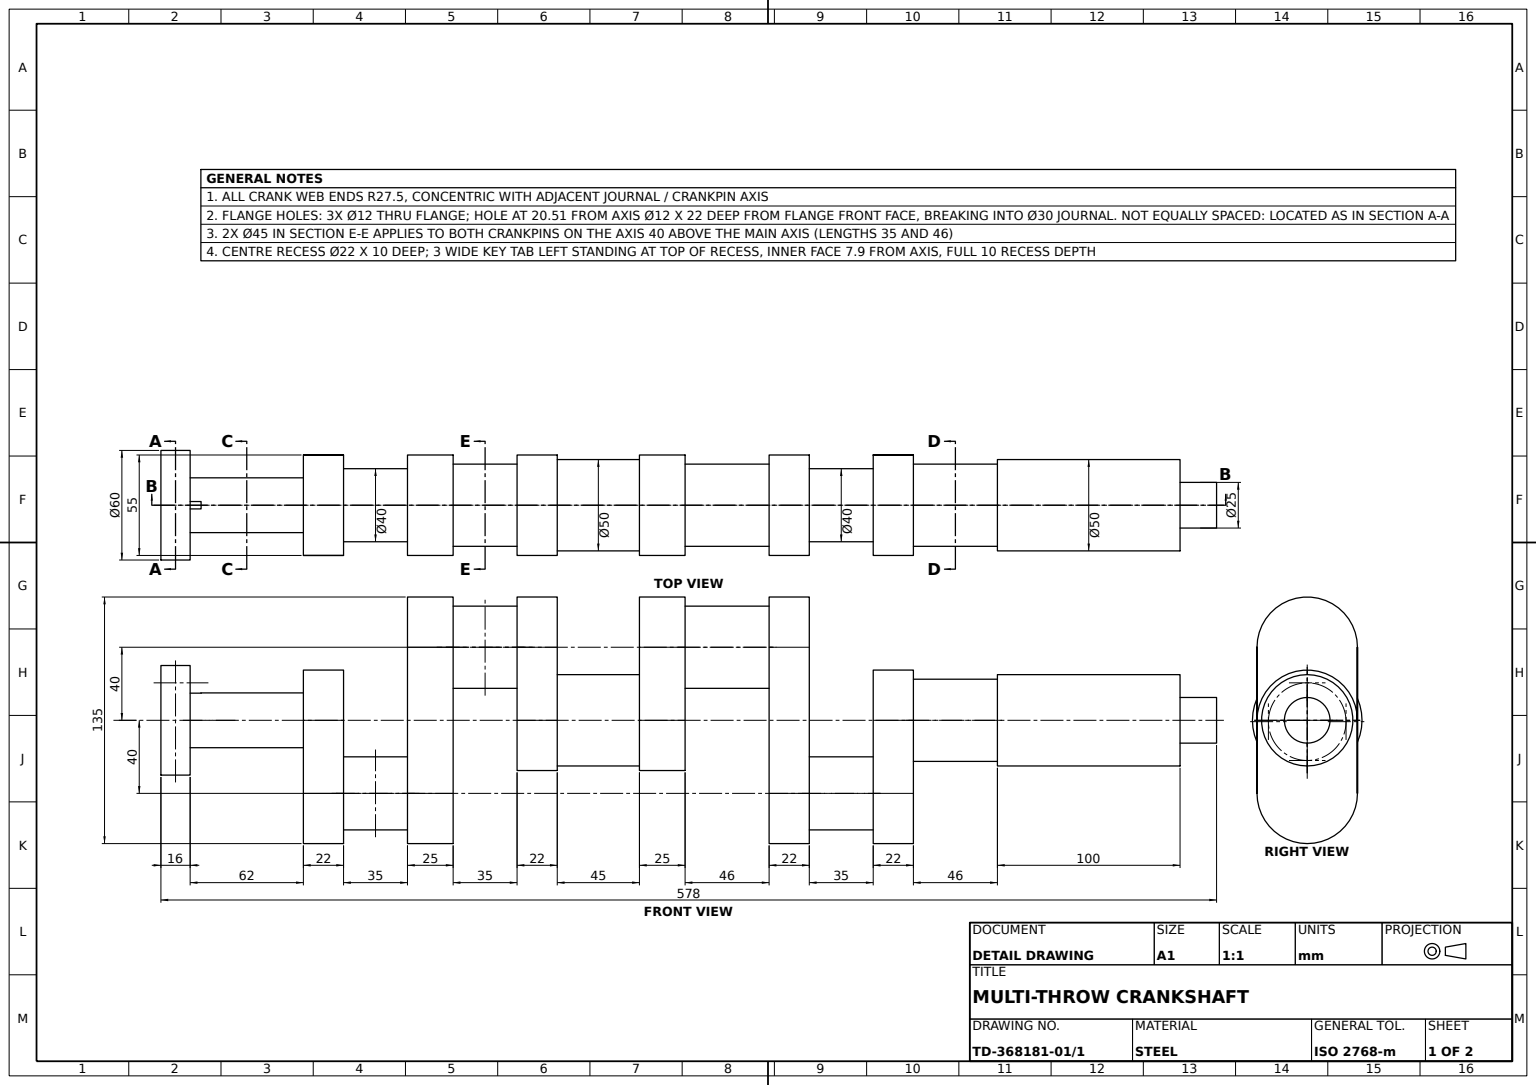
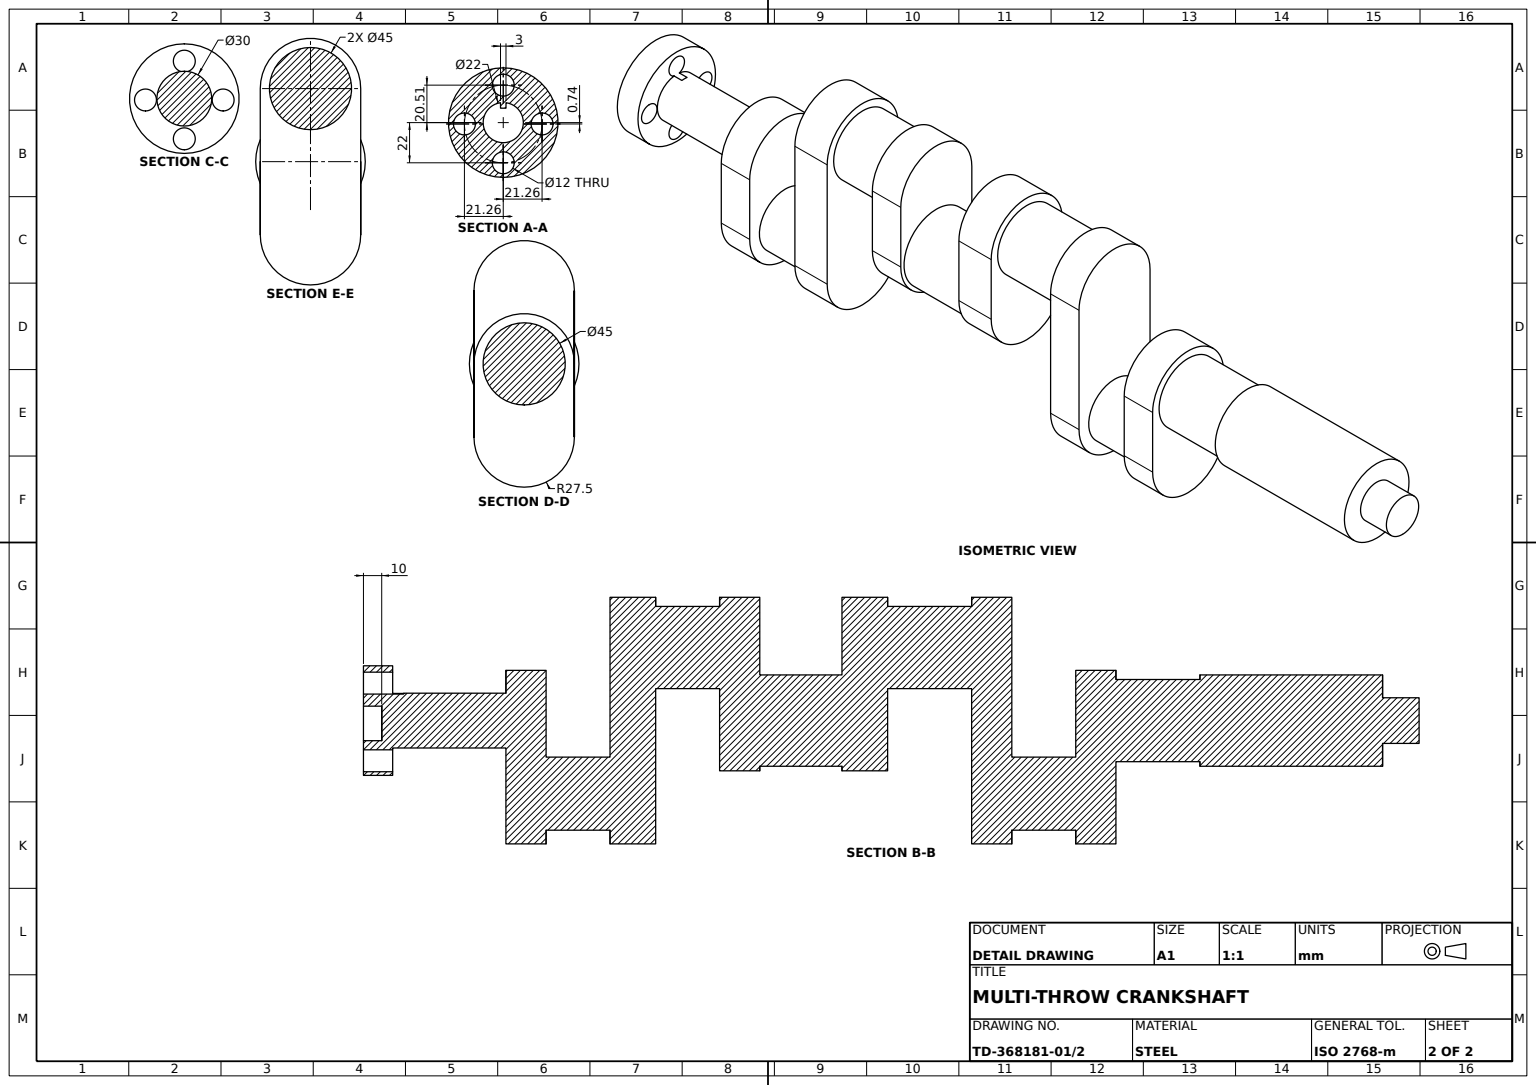
solid
v1 (-40,-27.5,-317)
v2 (-40,27.5,-317)
e1 v1 v2 CIRCLE(AX(P(-40,0,-317),D(0,0,-1),D(-1,0,0)),27.5)
v3 (-40,27.5,-339)
e2 v3 v2 LINE
v4 (-40,-27.5,-339)
e3 v4 v3 CIRCLE(AX(P(-40,0,-339),D(0,0,-1),D(-1,0,0)),27.5)
e4 v4 v1 LINE
face CYL(AX(P(-40,0,-339),D(0,0,1),D(1,0,0)),27.5) [e1 -e2 -e3 e4]
v5 (20,0,-84)
v6 (60,0,-84)
e5 v5 v6 CIRCLE(AX(P(40,0,-84),D(0,0,-1),D(-1,0,0)),20)
e6 v6 v5 CIRCLE(AX(P(40,0,-84),D(0,0,-1),D(-1,0,0)),20)
v7 (0,27.5,-84)
v8 (40,27.5,-84)
e7 v7 v8 LINE
v9 (67.5,0,-84)
e8 v8 v9 CIRCLE(AX(P(40,0,-84),D(0,0,-1),D(-1,0,0)),27.5)
v10 (40,-27.5,-84)
e9 v9 v10 CIRCLE(AX(P(40,0,-84),D(0,0,-1),D(-1,0,0)),27.5)
v11 (0,-27.5,-84)
e10 v10 v11 LINE
e11 v11 v7 CIRCLE(AX(P(0,0,-84),D(0,0,-1),D(-1,0,0)),27.5)
face PLANE(AX(P(0,0,-84),D(0,0,-1),D(-1,0,0))) [-e5 -e6] [e7 e8 e9 e10 e11]
v12 (25,0,-246)
v13 (-25,0,-246)
e12 v12 v13 CIRCLE(AX(P(0,0,-246),D(0,0,-1),D(-1,0,0)),25)
v14 (25,0,-201)
e13 v14 v12 LINE
v15 (-25,0,-201)
e14 v14 v15 CIRCLE(AX(P(0,0,-201),D(0,0,-1),D(-1,0,0)),25)
e15 v15 v13 LINE
face CYL(AX(P(0,0,-261.1485851),D(0,0,-1),D(-1,0,0)),25) [-e12 -e13 e14 e15]
v16 (16,0,0)
v17 (16,0,16)
e16 v16 v17 LINE
v18 (28,0,16)
e17 v17 v18 CIRCLE(AX(P(22,0,16),D(0,0,1),D(1,0,0)),6)
v19 (28,0,0)
e18 v19 v18 LINE
e19 v16 v19 CIRCLE(AX(P(22,0,0),D(0,0,1),D(1,0,0)),6)
face CYL(AX(P(22,0,-6),D(0,0,1),D(1,0,0)),6) rev [e16 e17 -e18 -e19]
v20 (-40,-27.5,-144)
v21 (-40,-27.5,-119)
e20 v20 v21 LINE
v22 (40,-27.5,-144)
e21 v22 v20 LINE
v23 (40,-27.5,-119)
e22 v22 v23 LINE
e23 v23 v21 LINE
face PLANE(AX(P(40,-27.5,-144),D(0,1,0),D(0,0,1))) rev [-e20 -e21 e22 e23]
v24 (25,0,-442)
v25 (-25,0,-442)
e24 v24 v25 CIRCLE(AX(P(0,0,-442),D(0,0,1),D(1,0,0)),25)
e25 v25 v24 CIRCLE(AX(P(0,0,-442),D(0,0,1),D(1,0,0)),25)
v26 (-22.5,0,-442)
v27 (22.5,0,-442)
e26 v26 v27 CIRCLE(AX(P(0,0,-442),D(0,0,1),D(1,0,0)),22.5)
e27 v27 v26 CIRCLE(AX(P(0,0,-442),D(0,0,1),D(1,0,0)),22.5)
face PLANE(AX(P(0,0,-442),D(0,0,1),D(1,0,0))) [e24 e25] [-e26 -e27]
v28 (-40,-27.5,-271)
v29 (-40,-27.5,-246)
e28 v28 v29 LINE
v30 (0,-27.5,-271)
e29 v30 v28 LINE
v31 (0,-27.5,-246)
e30 v30 v31 LINE
e31 v31 v29 LINE
face PLANE(AX(P(0,-27.5,-271),D(0,1,0),D(0,0,1))) rev [-e28 -e29 e30 e31]
v32 (-12.5,0,-562)
v33 (-12.5,0,-542)
e32 v32 v33 LINE
v34 (12.5,0,-562)
e33 v32 v34 CIRCLE(AX(P(0,0,-562),D(0,0,1),D(1,0,0)),12.5)
v35 (12.5,0,-542)
e34 v34 v35 LINE
e35 v33 v35 CIRCLE(AX(P(0,0,-542),D(0,0,1),D(1,0,0)),12.5)
face CYL(AX(P(0,0,-542),D(0,0,1),D(1,0,0)),12.5) [-e32 e33 e34 -e35]
v36 (6.7437452,-21.2562548,0)
v37 (6.7437452,-21.2562548,16)
e36 v36 v37 LINE
v38 (-5.2562548,-21.2562548,16)
e37 v37 v38 CIRCLE(AX(P(0.7437452,-21.2562548,16),D(0,0,1),D(1,0,0)),6)
v39 (-5.2562548,-21.2562548,0)
e38 v39 v38 LINE
e39 v36 v39 CIRCLE(AX(P(0.7437452,-21.2562548,0),D(0,0,1),D(1,0,0)),6)
face CYL(AX(P(0.7437452,-21.2562548,-6),D(0,0,1),D(1,0,0)),6) rev [e36 e37 -e38 -e39]
v40 (-15,0,-6)
v41 (-14.8631996,-2.0212116,-6)
e40 v40 v41 CIRCLE(AX(P(0,0,-6),D(0,0,1),D(1,0,0)),15)
v42 (-15,0,-62)
e41 v40 v42 LINE
v43 (15,0,-62)
e42 v43 v42 CIRCLE(AX(P(0,0,-62),D(0,0,-1),D(-1,0,0)),15)
v44 (15,0,0)
e43 v44 v43 LINE
v45 (-14.8631996,-2.0212116,0)
e44 v44 v45 CIRCLE(AX(P(0,0,0),D(0,0,-1),D(-1,0,0)),15)
e45 v45 v41 LINE
face CYL(AX(P(0,0,-63.5307628),D(0,0,-1),D(-1,0,0)),15) [-e40 e41 -e42 -e43 e44 e45]
e46 v39 v36 CIRCLE(AX(P(0.7437452,-21.2562548,0),D(0,0,1),D(1,0,0)),6)
e47 v38 v37 CIRCLE(AX(P(0.7437452,-21.2562548,16),D(0,0,1),D(1,0,0)),6)
face CYL(AX(P(0.7437452,-21.2562548,-6),D(0,0,1),D(1,0,0)),6) rev [-e46 e38 e47 -e36]
v46 (-26.5125097,0,0)
v47 (-26.5125097,0,16)
e48 v46 v47 LINE
v48 (-14.5125097,0,16)
e49 v47 v48 CIRCLE(AX(P(-20.5125097,0,16),D(0,0,1),D(1,0,0)),6)
v49 (-14.5125097,0,-6)
e50 v49 v48 LINE
e51 v41 v49 CIRCLE(AX(P(-20.5125097,0,-6),D(0,0,1),D(1,0,0)),6)
e52 v46 v45 CIRCLE(AX(P(-20.5125097,0,0),D(0,0,1),D(1,0,0)),6)
face CYL(AX(P(-20.5125097,0,-6),D(0,0,1),D(1,0,0)),6) rev [e48 e49 -e50 -e51 -e45 -e52]
v50 (40,27.5,-317)
v51 (67.5,0,-317)
e53 v50 v51 CIRCLE(AX(P(40,0,-317),D(0,0,-1),D(-1,0,0)),27.5)
v52 (67.5,0,-339)
e54 v52 v51 LINE
v53 (40,27.5,-339)
e55 v53 v52 CIRCLE(AX(P(40,0,-339),D(0,0,-1),D(-1,0,0)),27.5)
e56 v53 v50 LINE
face CYL(AX(P(40,0,-339),D(0,0,1),D(1,0,0)),27.5) [e53 -e54 -e55 e56]
v54 (-7.8972474,1.5,6)
v55 (-7.8972474,1.5,16)
e57 v54 v55 LINE
v56 (-7.8972474,-1.5,16)
e58 v55 v56 LINE
v57 (-7.8972474,-1.5,6)
e59 v57 v56 LINE
e60 v54 v57 LINE
face PLANE(AX(P(-7.8972474,1.5,6),D(-1,0,0),D(0,0,1))) rev [e57 e58 -e59 -e60]
v58 (-10.8972474,-1.5,6)
v59 (-10.8972474,-1.5,16)
e61 v58 v59 LINE
v60 (11,0,16)
e62 v59 v60 CIRCLE(AX(P(0,0,16),D(0,0,1),D(1,0,0)),11)
v61 (11,0,6)
e63 v61 v60 LINE
e64 v58 v61 CIRCLE(AX(P(0,0,6),D(0,0,1),D(1,0,0)),11)
face CYL(AX(P(0,0,6),D(0,0,1),D(1,0,0)),11) rev [e61 e62 -e63 -e64]
v62 (67.5,0,-396)
v63 (40,-27.5,-396)
e65 v62 v63 CIRCLE(AX(P(40,0,-396),D(0,0,-1),D(-1,0,0)),27.5)
v64 (67.5,0,-374)
e66 v62 v64 LINE
v65 (40,-27.5,-374)
e67 v64 v65 CIRCLE(AX(P(40,0,-374),D(0,0,-1),D(-1,0,0)),27.5)
e68 v63 v65 LINE
face CYL(AX(P(40,0,-396),D(0,0,1),D(1,0,0)),27.5) [-e65 e66 e67 -e68]
v66 (0,27.5,-62)
v67 (40,27.5,-62)
e69 v66 v67 LINE
e70 v8 v67 LINE
e71 v7 v66 LINE
face PLANE(AX(P(40,27.5,-84),D(0,-1,0),D(1,0,0))) rev [e69 -e70 -e7 e71]
v68 (20,0,-339)
v69 (60,0,-339)
e72 v68 v69 CIRCLE(AX(P(40,0,-339),D(0,0,-1),D(-1,0,0)),20)
e73 v69 v68 CIRCLE(AX(P(40,0,-339),D(0,0,-1),D(-1,0,0)),20)
e74 v3 v53 LINE
v70 (40,-27.5,-339)
e75 v52 v70 CIRCLE(AX(P(40,0,-339),D(0,0,-1),D(-1,0,0)),27.5)
e76 v70 v4 LINE
face PLANE(AX(P(40,0,-339),D(0,0,-1),D(-1,0,0))) [-e72 -e73] [e74 e55 e75 e76 e3]
v71 (-40,27.5,-144)
v72 (-40,27.5,-119)
e77 v71 v72 LINE
e78 v20 v71 CIRCLE(AX(P(-40,0,-144),D(0,0,-1),D(-1,0,0)),27.5)
e79 v21 v72 CIRCLE(AX(P(-40,0,-119),D(0,0,-1),D(-1,0,0)),27.5)
face CYL(AX(P(-40,0,-144),D(0,0,1),D(1,0,0)),27.5) [-e77 -e78 e20 e79]
e80 v35 v33 CIRCLE(AX(P(0,0,-542),D(0,0,1),D(1,0,0)),12.5)
e81 v34 v32 CIRCLE(AX(P(0,0,-562),D(0,0,1),D(1,0,0)),12.5)
face CYL(AX(P(0,0,-542),D(0,0,1),D(1,0,0)),12.5) [-e80 -e34 e81 e32]
v73 (0,27.5,-271)
v74 (27.5,0,-271)
e82 v73 v74 CIRCLE(AX(P(0,0,-271),D(0,0,-1),D(-1,0,0)),27.5)
e83 v74 v30 CIRCLE(AX(P(0,0,-271),D(0,0,-1),D(-1,0,0)),27.5)
v75 (-40,27.5,-271)
e84 v28 v75 CIRCLE(AX(P(-40,0,-271),D(0,0,-1),D(-1,0,0)),27.5)
e85 v73 v75 LINE
v76 (-17.5,0,-271)
v77 (-62.5,0,-271)
e86 v76 v77 CIRCLE(AX(P(-40,0,-271),D(0,0,-1),D(-1,0,0)),22.5)
e87 v77 v76 CIRCLE(AX(P(-40,0,-271),D(0,0,-1),D(-1,0,0)),22.5)
face PLANE(AX(P(0,0,-271),D(0,0,-1),D(-1,0,0))) [e82 e83 e29 e84 -e85] [-e86 -e87]
v78 (0,-27.5,-396)
v79 (0,-27.5,-374)
e88 v78 v79 LINE
e89 v63 v78 LINE
e90 v65 v79 LINE
face PLANE(AX(P(0,-27.5,-396),D(0,1,0),D(-1,0,0))) rev [-e88 -e89 e68 e90]
v80 (-17.5,0,-317)
e91 v80 v76 LINE
v81 (-62.5,0,-317)
e92 v80 v81 CIRCLE(AX(P(-40,0,-317),D(0,0,1),D(1,0,0)),22.5)
e93 v81 v77 LINE
face CYL(AX(P(-40,0,-271),D(0,0,1),D(1,0,0)),22.5) [e87 -e91 e92 e93]
e94 v19 v16 CIRCLE(AX(P(22,0,0),D(0,0,1),D(1,0,0)),6)
e95 v18 v17 CIRCLE(AX(P(22,0,16),D(0,0,1),D(1,0,0)),6)
face CYL(AX(P(22,0,-6),D(0,0,1),D(1,0,0)),6) rev [-e94 e18 e95 -e16]
v82 (-40,27.5,-246)
e96 v75 v82 LINE
e97 v29 v82 CIRCLE(AX(P(-40,0,-246),D(0,0,-1),D(-1,0,0)),27.5)
face CYL(AX(P(-40,0,-271),D(0,0,1),D(1,0,0)),27.5) [-e96 -e84 e28 e97]
v83 (-10.8972474,1.5,6)
e98 v61 v83 CIRCLE(AX(P(0,0,6),D(0,0,1),D(1,0,0)),11)
v84 (-10.8972474,1.5,16)
e99 v60 v84 CIRCLE(AX(P(0,0,16),D(0,0,1),D(1,0,0)),11)
e100 v83 v84 LINE
face CYL(AX(P(0,0,6),D(0,0,1),D(1,0,0)),11) rev [-e98 e63 e99 -e100]
v85 (-40,27.5,-201)
v86 (0,27.5,-201)
e101 v85 v86 LINE
v87 (-40,27.5,-179)
e102 v85 v87 LINE
v88 (0,27.5,-179)
e103 v87 v88 LINE
e104 v86 v88 LINE
face PLANE(AX(P(0,27.5,-201),D(0,-1,0),D(0,0,-1))) rev [-e101 e102 e103 -e104]
e105 v81 v80 CIRCLE(AX(P(-40,0,-317),D(0,0,1),D(1,0,0)),22.5)
v89 (40,-27.5,-317)
e106 v51 v89 CIRCLE(AX(P(40,0,-317),D(0,0,-1),D(-1,0,0)),27.5)
e107 v2 v50 LINE
e108 v89 v1 LINE
face PLANE(AX(P(40,0,-317),D(0,0,-1),D(-1,0,0))) rev [-e105 -e92] [-e106 -e53 -e107 -e1 -e108]
v90 (25,0,-542)
e109 v90 v24 LINE
v91 (-25,0,-542)
e110 v90 v91 CIRCLE(AX(P(0,0,-542),D(0,0,1),D(1,0,0)),25)
e111 v91 v25 LINE
face CYL(AX(P(0,0,-442),D(0,0,1),D(1,0,0)),25) [-e24 -e109 e110 e111]
e112 v91 v90 CIRCLE(AX(P(0,0,-542),D(0,0,1),D(1,0,0)),25)
face CYL(AX(P(0,0,-442),D(0,0,1),D(1,0,0)),25) [e109 -e25 -e111 e112]
v92 (0,-27.5,-62)
e113 v92 v66 CIRCLE(AX(P(0,0,-62),D(0,0,-1),D(-1,0,0)),27.5)
e114 v11 v92 LINE
face CYL(AX(P(0,0,-84),D(0,0,1),D(1,0,0)),27.5) [e113 -e71 -e11 e114]
v93 (40,-27.5,-62)
e115 v93 v92 LINE
v94 (67.5,0,-62)
e116 v94 v93 CIRCLE(AX(P(40,0,-62),D(0,0,-1),D(-1,0,0)),27.5)
e117 v67 v94 CIRCLE(AX(P(40,0,-62),D(0,0,-1),D(-1,0,0)),27.5)
e118 v42 v43 CIRCLE(AX(P(0,0,-62),D(0,0,-1),D(-1,0,0)),15)
face PLANE(AX(P(0,0,-62),D(0,0,-1),D(-1,0,0))) rev [-e69 -e113 -e115 -e116 -e117] [e118 e42]
face PLANE(AX(P(0,0,-542),D(0,0,-1),D(-1,0,0))) [e80 e35] [-e112 -e110]
e119 v10 v93 LINE
face PLANE(AX(P(40,-27.5,-84),D(0,1,0),D(-1,0,0))) rev [e115 -e114 -e10 e119]
v95 (-14.8631996,2.0212116,0)
e120 v95 v44 CIRCLE(AX(P(0,0,0),D(0,0,-1),D(-1,0,0)),15)
v96 (-14.8631996,2.0212116,-6)
e121 v96 v40 CIRCLE(AX(P(0,0,-6),D(0,0,1),D(1,0,0)),15)
e122 v96 v95 LINE
face CYL(AX(P(0,0,-63.5307628),D(0,0,-1),D(-1,0,0)),15) [e120 e43 -e118 -e41 -e121 e122]
e123 v15 v14 CIRCLE(AX(P(0,0,-201),D(0,0,-1),D(-1,0,0)),25)
v97 (27.5,0,-201)
e124 v86 v97 CIRCLE(AX(P(0,0,-201),D(0,0,-1),D(-1,0,0)),27.5)
v98 (0,-27.5,-201)
e125 v97 v98 CIRCLE(AX(P(0,0,-201),D(0,0,-1),D(-1,0,0)),27.5)
v99 (-40,-27.5,-201)
e126 v98 v99 LINE
e127 v99 v85 CIRCLE(AX(P(-40,0,-201),D(0,0,-1),D(-1,0,0)),27.5)
face PLANE(AX(P(0,0,-201),D(0,0,-1),D(-1,0,0))) [-e14 -e123] [e124 e125 e126 e127 e101]
e128 v83 v54 LINE
e129 v57 v58 LINE
face PLANE(AX(P(0,0,6),D(0,0,1),D(1,0,0))) [e98 e128 e60 e129 e64]
v100 (6.7437452,21.2562548,0)
v101 (-5.2562548,21.2562548,0)
e130 v100 v101 CIRCLE(AX(P(0.7437452,21.2562548,0),D(0,0,1),D(1,0,0)),6)
v102 (6.7437452,21.2562548,16)
e131 v100 v102 LINE
v103 (-5.2562548,21.2562548,16)
e132 v102 v103 CIRCLE(AX(P(0.7437452,21.2562548,16),D(0,0,1),D(1,0,0)),6)
e133 v101 v103 LINE
face CYL(AX(P(0.7437452,21.2562548,-6),D(0,0,1),D(1,0,0)),6) rev [-e130 e131 e132 -e133]
e134 v56 v59 LINE
face PLANE(AX(P(-7.8972474,-1.5,6),D(0,1,0),D(-1,0,0))) rev [e59 e134 -e61 -e129]
v104 (40,27.5,-374)
e135 v104 v64 CIRCLE(AX(P(40,0,-374),D(0,0,-1),D(-1,0,0)),27.5)
v105 (0,27.5,-374)
e136 v104 v105 LINE
e137 v79 v105 CIRCLE(AX(P(0,0,-374),D(0,0,-1),D(-1,0,0)),27.5)
v106 (20,0,-374)
v107 (60,0,-374)
e138 v106 v107 CIRCLE(AX(P(40,0,-374),D(0,0,1),D(1,0,0)),20)
e139 v107 v106 CIRCLE(AX(P(40,0,-374),D(0,0,1),D(1,0,0)),20)
face PLANE(AX(P(0,0,-374),D(0,0,-1),D(-1,0,0))) rev [-e67 -e135 e136 -e137 -e90] [-e138 -e139]
v108 (40,27.5,-144)
e140 v71 v108 LINE
v109 (67.5,0,-144)
e141 v108 v109 CIRCLE(AX(P(40,0,-144),D(0,0,-1),D(-1,0,0)),27.5)
e142 v109 v22 CIRCLE(AX(P(40,0,-144),D(0,0,-1),D(-1,0,0)),27.5)
v110 (-62.5,0,-144)
v111 (-17.5,0,-144)
e143 v110 v111 CIRCLE(AX(P(-40,0,-144),D(0,0,-1),D(-1,0,0)),22.5)
e144 v111 v110 CIRCLE(AX(P(-40,0,-144),D(0,0,-1),D(-1,0,0)),22.5)
face PLANE(AX(P(40,0,-144),D(0,0,-1),D(-1,0,0))) [e21 e78 e140 e141 e142] [-e143 -e144]
v112 (27.5,0,-246)
e145 v74 v112 LINE
e146 v112 v31 CIRCLE(AX(P(0,0,-246),D(0,0,-1),D(-1,0,0)),27.5)
face CYL(AX(P(0,0,-271),D(0,0,1),D(1,0,0)),27.5) [e145 e146 -e30 -e83]
e147 v103 v102 CIRCLE(AX(P(0.7437452,21.2562548,16),D(0,0,1),D(1,0,0)),6)
e148 v101 v100 CIRCLE(AX(P(0.7437452,21.2562548,0),D(0,0,1),D(1,0,0)),6)
face CYL(AX(P(0.7437452,21.2562548,-6),D(0,0,1),D(1,0,0)),6) rev [e133 e147 -e131 -e148]
face PLANE(AX(P(12.5,0,-562),D(0,0,-1),D(-1,0,0))) [-e81 -e33]
e149 v9 v94 LINE
face CYL(AX(P(40,0,-84),D(0,0,1),D(1,0,0)),27.5) [-e149 -e8 e70 e117]
e150 v70 v89 LINE
face CYL(AX(P(40,0,-339),D(0,0,1),D(1,0,0)),27.5) [-e75 e54 e106 -e150]
v113 (-17.5,0,-179)
v114 (-62.5,0,-179)
e151 v113 v114 CIRCLE(AX(P(-40,0,-179),D(0,0,1),D(1,0,0)),22.5)
e152 v114 v110 LINE
e153 v113 v111 LINE
face CYL(AX(P(-40,0,-144),D(0,0,1),D(1,0,0)),22.5) [e151 e152 e143 -e153]
e154 v13 v12 CIRCLE(AX(P(0,0,-246),D(0,0,-1),D(-1,0,0)),25)
face CYL(AX(P(0,0,-261.1485851),D(0,0,-1),D(-1,0,0)),25) [e13 -e154 -e15 e123]
v115 (40,27.5,-396)
e155 v115 v62 CIRCLE(AX(P(40,0,-396),D(0,0,-1),D(-1,0,0)),27.5)
e156 v115 v104 LINE
face CYL(AX(P(40,0,-396),D(0,0,1),D(1,0,0)),27.5) [-e66 -e155 e156 e135]
v116 (-40,-27.5,-179)
e157 v99 v116 LINE
v117 (0,-27.5,-179)
e158 v98 v117 LINE
e159 v117 v116 LINE
face PLANE(AX(P(0,-27.5,-201),D(0,1,0),D(0,0,1))) rev [-e157 -e126 e158 e159]
v118 (27.5,0,-179)
e160 v97 v118 LINE
e161 v118 v117 CIRCLE(AX(P(0,0,-179),D(0,0,-1),D(-1,0,0)),27.5)
face CYL(AX(P(0,0,-201),D(0,0,1),D(1,0,0)),27.5) [-e125 e160 e161 -e158]
v119 (60,0,-119)
e162 v119 v6 LINE
v120 (20,0,-119)
e163 v120 v5 LINE
e164 v120 v119 CIRCLE(AX(P(40,0,-119),D(0,0,1),D(1,0,0)),20)
face CYL(AX(P(40,0,-84),D(0,0,1),D(1,0,0)),20) [e162 e6 -e163 e164]
face CYL(AX(P(-40,0,-271),D(0,0,1),D(1,0,0)),22.5) [e105 e91 e86 -e93]
e165 v116 v87 CIRCLE(AX(P(-40,0,-179),D(0,0,-1),D(-1,0,0)),27.5)
face CYL(AX(P(-40,0,-201),D(0,0,1),D(1,0,0)),27.5) [-e127 e157 e165 -e102]
v121 (40,27.5,-119)
e166 v108 v121 LINE
e167 v72 v121 LINE
face PLANE(AX(P(40,27.5,-144),D(0,-1,0),D(0,0,-1))) rev [-e166 -e140 e77 e167]
v122 (67.5,0,-119)
e168 v122 v23 CIRCLE(AX(P(40,0,-119),D(0,0,-1),D(-1,0,0)),27.5)
e169 v109 v122 LINE
face CYL(AX(P(40,0,-144),D(0,0,1),D(1,0,0)),27.5) [e168 -e22 -e142 e169]
v123 (0,27.5,-246)
e170 v123 v112 CIRCLE(AX(P(0,0,-246),D(0,0,-1),D(-1,0,0)),27.5)
e171 v123 v82 LINE
face PLANE(AX(P(0,0,-246),D(0,0,-1),D(-1,0,0))) rev [e154 e12] [-e31 -e146 -e170 e171 -e97]
v124 (30,0,16)
v125 (-30,0,16)
e172 v124 v125 CIRCLE(AX(P(0,0,16),D(0,0,1),D(1,0,0)),30)
v126 (30,0,0)
e173 v124 v126 LINE
v127 (-30,0,0)
e174 v126 v127 CIRCLE(AX(P(0,0,0),D(0,0,1),D(1,0,0)),30)
e175 v125 v127 LINE
face CYL(AX(P(0,0,16),D(0,0,-1),D(-1,0,0)),30) [-e172 e173 e174 -e175]
e176 v84 v55 LINE
face PLANE(AX(P(-10.8972474,1.5,6),D(0,-1,0),D(1,0,0))) rev [e176 -e57 -e128 e100]
e177 v114 v113 CIRCLE(AX(P(-40,0,-179),D(0,0,1),D(1,0,0)),22.5)
e178 v88 v118 CIRCLE(AX(P(0,0,-179),D(0,0,-1),D(-1,0,0)),27.5)
face PLANE(AX(P(0,0,-179),D(0,0,-1),D(-1,0,0))) rev [-e177 -e151] [-e178 -e103 -e165 -e159 -e161]
e179 v127 v126 CIRCLE(AX(P(0,0,0),D(0,0,1),D(1,0,0)),30)
e180 v95 v46 CIRCLE(AX(P(-20.5125097,0,0),D(0,0,1),D(1,0,0)),6)
face PLANE(AX(P(0,0,0),D(0,0,1),D(1,0,0))) rev [e19 e94] [e39 e46] [e148 e130] [-e174 -e179] [e180 e52 -e44 -e120]
e181 v106 v68 LINE
e182 v107 v69 LINE
face CYL(AX(P(40,0,-339),D(0,0,1),D(1,0,0)),20) [e73 -e181 e138 e182]
face CYL(AX(P(40,0,-84),D(0,0,1),D(1,0,0)),27.5) [-e119 -e9 e149 e116]
e183 v73 v123 LINE
face PLANE(AX(P(0,27.5,-271),D(0,1,0),D(0,0,1))) [e96 -e171 -e183 e85]
e184 v121 v122 CIRCLE(AX(P(40,0,-119),D(0,0,-1),D(-1,0,0)),27.5)
face CYL(AX(P(40,0,-144),D(0,0,1),D(1,0,0)),27.5) [e184 -e169 -e141 e166]
face CYL(AX(P(0,0,-271),D(0,0,1),D(1,0,0)),27.5) [e183 e170 -e145 -e82]
v128 (-22.5,0,-396)
e185 v26 v128 LINE
v129 (22.5,0,-396)
e186 v129 v128 CIRCLE(AX(P(0,0,-396),D(0,0,1),D(1,0,0)),22.5)
e187 v27 v129 LINE
face CYL(AX(P(0,0,-396),D(0,0,1),D(1,0,0)),22.5) [e27 e185 -e186 -e187]
e188 v48 v47 CIRCLE(AX(P(-20.5125097,0,16),D(0,0,1),D(1,0,0)),6)
e189 v125 v124 CIRCLE(AX(P(0,0,16),D(0,0,1),D(1,0,0)),30)
face PLANE(AX(P(0,0,16),D(0,0,1),D(1,0,0))) [-e95 -e17] [-e188 -e49] [-e134 -e58 -e176 -e99 -e62] [-e37 -e47] [e189 e172] [-e132 -e147]
face PLANE(AX(P(40,27.5,-339),D(0,-1,0),D(1,0,0))) rev [-e74 e2 e107 -e56]
v130 (0,27.5,-396)
e190 v130 v105 LINE
e191 v78 v130 CIRCLE(AX(P(0,0,-396),D(0,0,-1),D(-1,0,0)),27.5)
face CYL(AX(P(0,0,-396),D(0,0,1),D(1,0,0)),27.5) [e88 e137 -e190 -e191]
e192 v119 v120 CIRCLE(AX(P(40,0,-119),D(0,0,1),D(1,0,0)),20)
face CYL(AX(P(40,0,-84),D(0,0,1),D(1,0,0)),20) [e163 e5 -e162 e192]
e193 v49 v96 CIRCLE(AX(P(-20.5125097,0,-6),D(0,0,1),D(1,0,0)),6)
face CYL(AX(P(-20.5125097,0,-6),D(0,0,1),D(1,0,0)),6) rev [e50 e188 -e48 -e180 -e122 -e193]
face CYL(AX(P(-40,0,-144),D(0,0,1),D(1,0,0)),22.5) [e144 -e152 e177 e153]
e194 v128 v129 CIRCLE(AX(P(0,0,-396),D(0,0,1),D(1,0,0)),22.5)
e195 v115 v130 LINE
face PLANE(AX(P(0,0,-396),D(0,0,-1),D(-1,0,0))) [e194 e186] [e191 -e195 e155 e65 e89]
face PLANE(AX(P(-20.5125097,0,-6),D(0,0,1),D(1,0,0))) [e121 e40 e51 e193]
face PLANE(AX(P(40,0,-119),D(0,0,-1),D(-1,0,0))) rev [-e79 -e23 -e168 -e184 -e167] [-e164 -e192]
face PLANE(AX(P(40,-27.5,-339),D(0,1,0),D(-1,0,0))) rev [e150 e108 -e4 -e76]
face PLANE(AX(P(0,27.5,-396),D(0,1,0),D(0,0,1))) [e190 -e136 -e156 e195]
face CYL(AX(P(0,0,-396),D(0,0,1),D(1,0,0)),22.5) [-e194 -e185 e26 e187]
face CYL(AX(P(0,0,-201),D(0,0,1),D(1,0,0)),27.5) [-e124 e104 e178 -e160]
face CYL(AX(P(40,0,-339),D(0,0,1),D(1,0,0)),20) [e139 e181 e72 -e182]
face CYL(AX(P(0,0,16),D(0,0,-1),D(-1,0,0)),30) [-e173 -e189 e175 e179]
